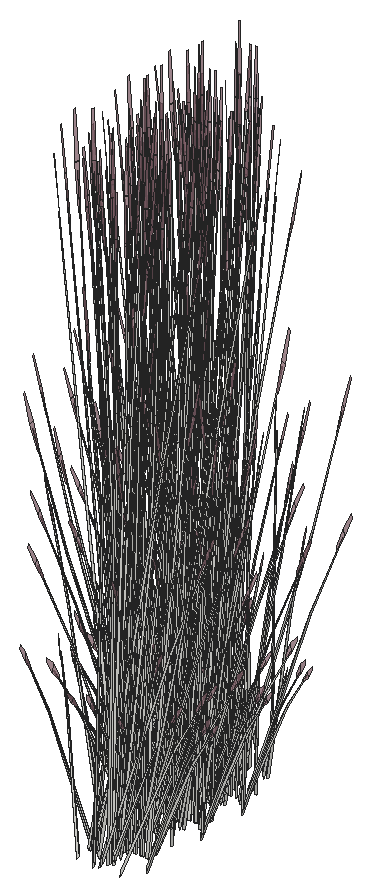
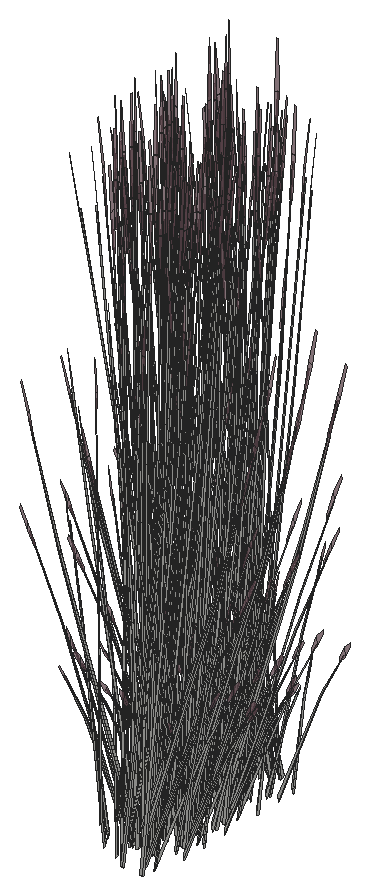
# SketchUp Ruby script. Lengths in inches.
U = 1.inch
M = Sketchup.active_model
def pt(a) = Geom::Point3d.new(a.map { |v| v * U })
def face(e, loops, mat)
  f = e.add_face(loops[0].map { |a| pt(a) })
  loops[1..].each { |l| e.add_face(l.map { |a| pt(a) }).erase! }
  f.material = f.back_material = mat if mat
  f
end
# faces: each face lists its corners as indices into pts; further lists are holes
def faces(e, pts, list, mat = nil) = list.each { |f| face(e, (f[0].is_a?(Array) ? f : [f]).map { |l| l.map { |i| pts[i] } }, mat) }
# xy, xz, yz: faces in a plane at the given z, y or x. An outline is a flat list of corners, or four numbers for a rectangle; further outlines are holes
def ring(l) = l.size == 4 ? [[l[0], l[1]], [l[2], l[1]], [l[2], l[3]], [l[0], l[3]]] : l.each_slice(2).to_a
def flat(e, list, mat, &to3) = list.each { |f| face(e, (f[0].is_a?(Array) ? f : [f]).map { |l| ring(l).map { |u, v| to3.(u, v) } }, mat) }
def xy(e, z, list, mat = nil) = flat(e, list, mat) { |x, y| [x, y, z] }
def xz(e, y, list, mat = nil) = flat(e, list, mat) { |x, z| [x, y, z] }
def yz(e, x, list, mat = nil) = flat(e, list, mat) { |y, z| [x, y, z] }
def lines(e, pts, list) = list.each { |a, b| e.add_line(pt(pts[a]), pt(pts[b])) }
# prism: a flat outline (further loops are holes) pulled along v
def prism(e, loops, v, mat = nil)
  f = face(e, loops, mat); d = Geom::Vector3d.new(v.map { |x| x * U })
  f.pushpull(f.normal.samedirection?(d) ? d.length : -d.length)
end
def box(e, o, s, mat = nil) = prism(e, [[o, [o[0] + s[0], o[1], o[2]], [o[0] + s[0], o[1] + s[1], o[2]], [o[0], o[1] + s[1], o[2]]]], [0, 0, s[2]], mat)
def at(x, y, z, deg = 0) = Geom::Transformation.translation(pt([x, y, z])) * Geom::Transformation.rotation(ORIGIN, Z_AXIS, deg.degrees)
def axes(o, x, y, z) = Geom::Transformation.new([*x, 0, *y, 0, *z, 0, *pt(o).to_a, 1])
def part(name) = M.definitions.add(name)
# library, detail: a bought-in or finely detailed component or shape, given as its bounding box
def library(name, o, s) = part(name).tap { |d| box(d.entities, o, s) }
def detail(e, o, s) = box(e.add_group.entities, o, s)
def put(e, d, t, mat = nil) = e.add_instance(d, t).tap { |i| i.material = mat if mat }
def group(e, t, mat = nil) = e.add_group.tap { |g| g.transformation = t; g.material = mat if mat }.entities
root = M.entities
M.materials.add("LightPink_Translucent").color = [144, 107, 117]
M.materials["LightPink_Translucent"].alpha = 0.75
c1 = part("blade")
p = [[2.15,0.21,22],[0,0.17,0],[0.09,0.45,0],[2.18,0.31,22],[2.29,0.31,22],[0.38,0.45,0],
  [2.48,0.24,33],[2.49,0.24,33],[2.48,0.22,33]]
faces(c1.entities,p,[[0,1,2,3],[4,5,2,3],[6,3,4,7],[8,0,3,6]])
c2 = part("seeds")
p = [[0.3,-0.1,1.38],[-0.01,-0.03,1.59],[-0.01,-0.03,0.03],[0.14,-0.07,-0.07],[0.29,-0.03,3],[0.15,0.01,3.11]]
faces(c2.entities,p,[[0,1,2,3],[1,0,4,5]],"LightPink_Translucent")
c3 = part("blade with seeds")
put(c3.entities,c1,at(0,0,0))
put(c3.entities,c2,axes([2.4,0.25,30.99],[1.5799,-0.05474,1.17369],[-0.12525,1.92788,0.29478],[-0.07173,-0.02425,1.56792]))
put(root,c3,axes([430.05,458.625,152.09],[-0.38354,-0.23583,0.41945],[0.22925,-0.42288,0],[0.08735,0.05371,1.33059]))
put(root,c3,axes([430.8,460.28,154.21],[0.3601,-0.20831,-0.60019],[0.20068,0.4288,0.07243],[0.17399,-0.04871,0.84903]))
put(root,c3,axes([429.18,459.54,151.99],[-0.33979,0.42804,0.38653],[-0.40368,-0.37784,0.15168],[0.08192,-0.04272,1.34202]))
put(root,c3,axes([429.56,460.31,151.94],[-0.38118,-0.40596,-0.0518],[0.38142,-0.40621,0],[-0.01331,-0.01418,1.48322]))
put(root,c3,axes([428.59,458.84,152.09],[-0.11838,0.46875,0.14904],[-0.43321,-0.13265,0.29641],[0.07483,-0.00228,1.35512]))
put(root,c3,axes([428.42,459.21,151.35],[-0.40337,0.18883,1.08919],[-0.12839,-0.54182,0.42321],[0.24769,0.00901,1.23883]))
put(root,c3,axes([429.5,459.36,152.21],[0.07906,-0.42093,0.12232],[0.38625,0.07307,-0.3493],[0.07029,0.04322,1.07074]))
put(root,c3,axes([429.76,458.01,151.97],[0.51304,0.1533,0.25983],[-0.12835,0.54797,-0.30828],[-0.08491,0.06858,1.39295]))
put(root,c3,axes([429.88,463.28,152.1875],[-0.11649,0.09547,1.20808],[-0.34886,-0.1671,-0.25981],[0.06467,-0.20781,0.51652]))
put(root,c3,axes([428.83,460.36,151.99],[0.51796,0.09937,0.38653],[-0.10541,0.56124,0.15168],[-0.07569,-0.05419,1.34202]))
put(root,c3,axes([431.57,459.95,151.26],[-0.02142,-0.07161,1.48974],[0.14855,-0.41887,-0.22758],[0.14984,-0.00603,0.25375]))
put(root,c3,axes([429.35,463.61,154.21],[-0.19559,-0.38351,-0.60019],[0.40262,-0.21373,0.07243],[-0.04574,-0.1853,0.84903]))
put(root,c3,axes([427.14,459.875,151.26],[0.01039,0.07433,1.48974],[-0.20952,0.38819,-0.22758],[-0.14882,-0.01957,0.25375]))
put(root,c3,axes([429.33,459.47,152.3],[-0.24618,-0.39589,0.37796],[0.37289,-0.27878,-0.1819],[0.07967,0.04899,1.2135]))
put(root,c3,axes([428.08,463.1,152.1875],[-0.02482,0.15429,1.20808],[-0.36278,0.12916,-0.25981],[-0.0848,-0.19943,0.51652]))
put(root,c3,axes([430.42,457.97,152.34],[-0.23074,-0.13562,0.97034],[0.29794,-0.1378,0.71294],[0.08036,0.11673,0.21373]))
put(root,c3,axes([429.02,462.76,151.26],[-0.06874,0.01699,1.48974],[-0.38012,-0.19128,-0.22758],[0.00638,-0.15955,0.25375]))
put(root,c3,axes([428.55,461.25,152.09],[0.44036,-0.12519,0.14904],[0.10874,0.46588,0.29641],[-0.03927,-0.06788,1.35512]))
put(root,c3,axes([429.46,459.49,152.25],[0.41376,-0.31314,-0.2458],[0.27514,0.44246,-0.42242],[0.10209,0.04493,1.34921]))
put(root,c3,axes([430.17,463.99,154.21],[0.01066,-0.43628,-0.60019],[0.44902,0.0293,0.07243],[0.04739,-0.18483,0.84903]))
put(root,c3,axes([429.78,460.01,151.86],[0.45849,0,0],[0,0.4883,0],[0,0,1.50718]))
put(root,c3,axes([430.08,458.31,152],[0.25622,0.47263,0],[-0.42866,0.26357,-0.43598],[-0.09763,0.06003,1.38303]))
put(root,c3,axes([429,460.62,152.25],[-0.41376,0.31314,-0.2458],[-0.27514,-0.44246,-0.42242],[-0.10209,-0.04493,1.34921]))
put(root,c3,axes([429.91,458.86,152.09],[-0.44036,0.12519,0.14904],[-0.10874,-0.46588,0.29641],[0.03927,0.06788,1.35512]))
put(root,c3,axes([430.48,458.47,151.26],[0.02986,-0.06809,1.48974],[0.37589,-0.20055,-0.22758],[0.11396,0.1038,0.25375]))
put(root,c3,axes([429.86,456.4375,152.4],[-0.01119,-0.44408,1.19347],[0.50665,0.11511,0.50532],[-0.11983,0.243,1.12654]))
put(root,c3,axes([427.03,458.41,151.26],[0.05497,0.04712,1.48974],[0.09321,0.43661,-0.22758],[-0.12183,0.0931,0.25375]))
put(root,c3,axes([429.46,462.52,152.34],[0.05257,0.27504,0.97034],[-0.29163,-0.15233,0.71294],[0.03138,-0.14083,0.21373]))
put(root,c3,axes([429.63,459.76,152.01],[-0.51796,-0.09937,0.41563],[0.10541,-0.56124,0.1631],[0.07569,0.05419,1.44303]))
put(root,c3,axes([430.46,458.58,152.25],[-0.26279,-0.01479,0.88755],[0.17355,-0.31417,0.49003],[0.10382,0.11162,0.6962]))
put(root,c3,axes([429.21,461.14,151.86],[-0.13371,-0.40664,0],[0.38182,-0.1424,0],[0,0,1.30413]))
put(root,c3,axes([428.96,460.76,152.21],[-0.07906,0.42093,0.12232],[-0.38625,-0.07307,-0.3493],[-0.07029,-0.04322,1.07074]))
put(root,c3,axes([429.71,461.09,151.85],[0.43024,-0.16003,-0.16218],[0.15118,0.46099,0.00007],[0.04749,-0.01769,1.46908]))
put(root,c3,axes([429.86,461.28,152.09],[0.11838,-0.46875,0.14904],[0.43321,0.13265,0.29641],[-0.07483,0.00228,1.35512]))
put(root,c3,axes([429.77,460.22,151.87],[0.28606,0.30466,0],[-0.28606,0.30466,0],[0,0,1.42996]))
put(root,c3,axes([430.54,460.08,152.09],[-0.32198,-0.34356,0.14904],[0.32447,-0.33323,0.29641],[-0.03556,0.07016,1.35512]))
put(root,c3,axes([427.96,462.85,152.34],[0.21377,0.16416,0.97034],[-0.31132,0.09868,0.71294],[-0.06661,-0.12616,0.21373]))
put(root,c3,axes([431.83,460.4,152.34],[-0.2532,0.07787,0.97034],[0.11918,-0.32181,0.71294],[0.13432,0.02202,0.21373]))
put(root,c3,axes([428.47,463.72,154.21],[-0.34944,-0.22798,-0.60019],[0.24834,-0.39949,0.07243],[-0.1266,-0.13612,0.84903]))
put(root,c3,axes([429.12,461.33,151.86],[-0.41314,-0.21175,0],[0.19883,-0.43999,0],[0,0,1.37455]))
put(root,c3,axes([429.46,460.76,152.08],[-0.40016,-0.37963,-0.21282],[0.33672,-0.42629,0.46574],[-0.10776,0.04441,1.42109]))
put(root,c3,axes([428.41,461.49,152.09],[0.38354,0.23583,0.41945],[-0.22925,0.42288,0],[-0.08735,-0.05371,1.33059]))
put(root,c3,axes([429.6,457.82,152.1875],[0.00723,-0.15635,1.20808],[0.34559,-0.17464,-0.25981],[0.10668,0.18713,0.51652]))
put(root,c3,axes([429.76,459.86,152.3],[0.19883,-0.425,0.37796],[0.41314,0.20454,-0.1819],[0,0.09797,1.2135]))
put(root,c3,axes([428.03,459.125,152.34],[-0.01061,-0.28045,0.97034],[0.26501,0.20003,0.71294],[-0.05212,0.13367,0.21373]))
put(root,c3,axes([429.68,460.1,151.9375],[0,0.54548,-0.04762],[-0.51243,0,0],[0,0.01714,1.5153]))
put(root,c3,axes([427.79,463.34,151.26],[-0.0397,0.06213,1.48974],[-0.40116,0.13396,-0.22758],[-0.09691,-0.12186,0.25375]))
put(root,c3,axes([428.1875,461.74,152],[-0.25622,0.47263,0],[-0.42866,-0.26357,-0.43598],[-0.09763,-0.06003,1.38303]))
put(root,c3,axes([428.73,458.45,151.26],[0.06632,-0.02567,1.48974],[0.39894,0.14126,-0.22758],[0.01167,0.15921,0.25375]))
put(root,c3,axes([430.8,460.1,152.09],[0,-0.47166,0.41945],[0.45849,0,0],[0,0.10742,1.33059]))
put(root,c3,axes([429.66,460.45,152.3],[0.44501,-0.02912,0.37796],[0.04024,0.48332,-0.1819],[-0.07967,0.04899,1.2135]))
put(root,c3,axes([430.7,463.57,151.26],[-0.06134,-0.03716,1.48974],[-0.15755,-0.41512,-0.22758],[0.10629,-0.11265,0.25375]))
put(root,c3,axes([429.93,459.96,152.21],[0.38182,-0.13755,0.12232],[0.13371,0.39278,-0.3493],[0,0.08644,1.07074]))
put(root,c3,axes([427.8125,458.52,152.38],[0.37228,-0.08352,0.05498],[0.08559,0.3365,-0.7291],[-0.0236,0.17034,0.65354]))
put(root,c3,axes([431.35,460.91,152.1875],[-0.0987,-0.116,1.20808],[0.12841,-0.38374,-0.25981],[0.19968,0.05198,0.51652]))
put(root,c3,axes([429.59,461.34,151.86],[0.41314,0.21175,0],[-0.19883,0.43999,0],[0,0,1.47801]))
put(root,c3,axes([430.7,464.74,154.21],[0.21406,-0.37215,-0.60019],[0.37511,0.26448,0.07243],[0.12781,-0.13483,0.84903]))
put(root,c3,axes([428.38,463.66,152],[-0.25622,-0.47263,0],[0.42866,-0.26357,-0.43598],[0.09763,-0.06003,1.38303]))
put(root,c3,axes([429.75,461.8,151.85],[-0.25302,-0.47428,-0.04344],[0.42866,-0.26357,0.43598],[-0.10563,0.04516,1.38235]))
put(root,c3,axes([428.95,463.09,151.8],[-0.28319,0.27058,-0.03288],[-0.25948,-0.29635,-0.1491],[-0.01827,-0.08397,0.4918]))
put(root,c3,axes([429.66,460.66,152.21],[0.30276,0.28338,0.12232],[-0.25254,0.31972,-0.3493],[-0.07029,0.04322,1.07074]))
put(root,c3,axes([430.45,461.15,154.21],[0.40965,0.01136,-0.60019],[-0.02751,0.47821,0.07243],[0.17355,0.05047,0.84903]))
put(root,c3,axes([428.85,458.27,154.21],[0.19559,0.38351,-0.60019],[-0.40262,0.21373,0.07243],[0.04574,0.1853,0.84903]))
put(root,c3,axes([429.99,461.53,152.09],[0.38354,-0.23583,0.41945],[0.22925,0.42288,0],[-0.08735,0.05371,1.33059]))
put(root,c3,axes([429.44,461.16,151.9375],[0.17817,0.54185,-0.05079],[-0.50909,0.18987,0],[0.00622,0.01892,1.45452]))
put(root,c3,axes([427.72,458.875,152.1875],[0.12932,-0.07441,1.20808],[0.31929,0.22435,-0.25981],[-0.09503,0.19413,0.51652]))
put(root,c3,axes([431.01,464.4,152.1875],[-0.1464,-0.01397,1.20808],[-0.14998,-0.37477,-0.25981],[0.17985,-0.10602,0.51652]))
put(root,c3,axes([426.88,460.91,152.1875],[0.14242,0.03872,1.20808],[0.09179,0.39548,-0.25981],[-0.19345,0.07403,0.51652]))
put(root,c3,axes([431.12,460.18,152.01],[0.51243,0,0],[0,0.52715,-0.43598],[0,0.12006,1.38303]))
put(root,c3,axes([430.91,460.45,151.86],[-0.51218,-0.00377,-0.04204],[0,-0.52715,0.42192],[-0.0161,0.12,1.33776]))
put(root,c3,axes([429.8,459.99,152.25],[0.46151,0.22505,-0.2458],[-0.22222,0.475,-0.42242],[0.0145,0.11662,1.34921]))
put(root,c3,axes([431.18,463.71,152.34],[-0.1365,0.2401,0.97034],[-0.11733,-0.32258,0.71294],[0.11274,-0.08083,0.21373]))
put(root,c3,axes([426.58,461.74,152.34],[0.17079,-0.21377,0.97034],[0.06739,0.33841,0.71294],[-0.12342,0.0606,0.21373]))
put(root,c3,axes([429.57,460.55,152.25],[0.04775,0.53819,-0.2458],[-0.49736,0.03254,-0.42242],[-0.08758,0.07169,1.34921]))
put(root,c3,axes([428.89,464.97,152.25],[-0.04775,-0.53819,-0.2458],[0.49736,-0.03254,-0.42242],[0.08758,-0.07169,1.34921]))
put(root,c3,axes([427.54,463.58,151.8],[-0.11822,0.38513,-0.03288],[-0.36385,-0.11847,-0.1491],[-0.05524,-0.06299,0.4918]))
put(root,c3,axes([428.66,465.53,152.25],[-0.46151,-0.22505,-0.2458],[0.22222,-0.475,-0.42242],[-0.0145,-0.11662,1.34921]))
put(root,c3,axes([427.34,465.34,152],[-0.51243,0,0],[0,-0.52715,-0.43598],[0,-0.12006,1.38303]))
put(root,c3,axes([427.43,464.4,152.1875],[0.08001,0.13132,1.20808],[-0.18437,0.35694,-0.25981],[-0.18931,-0.08532,0.51652]))
put(root,c3,axes([429.76,461.56,151.97],[0.51304,0.1533,0.25983],[-0.12835,0.54797,-0.30828],[-0.08491,0.06858,1.39295]))
put(root,c3,axes([427.76,464.28,154.21],[-0.40965,-0.01136,-0.60019],[0.02751,-0.47821,0.07243],[-0.17355,-0.05047,0.84903]))
put(root,c3,axes([430.42,461.51,152.34],[-0.23074,-0.13562,0.97034],[0.29794,-0.1378,0.71294],[0.08036,0.11673,0.21373]))
put(root,c3,axes([427.74,465.2,151.97],[-0.38118,0.39654,0.25983],[-0.38142,-0.39237,-0.30828],[-0.01331,-0.11261,1.39295]))
put(root,c3,axes([429.88,467.33,152.1875],[-0.11649,0.09547,1.20808],[-0.34886,-0.1671,-0.25981],[0.06467,-0.20781,0.51652]))
put(root,c3,axes([430.08,461.86,152],[0.25622,0.47263,0],[-0.42866,0.26357,-0.43598],[-0.09763,0.06003,1.38303]))
put(root,c3,axes([429.35,467.66,154.21],[-0.19559,-0.38351,-0.60019],[0.40262,-0.21373,0.07243],[-0.04574,-0.1853,0.84903]))
put(root,c3,axes([430.48,462.02,151.26],[0.02986,-0.06809,1.48974],[0.37589,-0.20055,-0.22758],[0.11396,0.1038,0.25375]))
put(root,c3,axes([429.86,459.99,152.4],[-0.01119,-0.44408,1.19347],[0.50665,0.11511,0.50532],[-0.11983,0.243,1.12654]))
put(root,c3,axes([428.08,467.15,152.1875],[-0.02482,0.15429,1.20808],[-0.36278,0.12916,-0.25981],[-0.0848,-0.19943,0.51652]))
put(root,c3,axes([427.03,461.96,151.26],[0.05497,0.04712,1.48974],[0.09321,0.43661,-0.22758],[-0.12183,0.0931,0.25375]))
put(root,c3,axes([428.95,465.39,152.06],[0.46174,0.2286,0.2033],[-0.22222,0.475,0.42242],[0,-0.1095,1.35626]))
put(root,c3,axes([428.77,466.03,152.06],[0.10862,-0.55889,-0.19793],[0.515,0.09742,0.43313],[-0.08999,-0.07718,1.32161]))
put(root,c3,axes([429.02,466.8125,151.26],[-0.06874,0.01699,1.48974],[-0.38012,-0.19128,-0.22758],[0.00638,-0.15955,0.25375]))
put(root,c3,axes([426.95,464.79,152.34],[0.26163,-0.03375,0.97034],[-0.16596,0.29737,0.71294],[-0.12929,-0.04461,0.21373]))
put(root,c3,axes([430.46,462.13,152.25],[-0.26279,-0.01479,0.88755],[0.17355,-0.31417,0.49003],[0.10382,0.11162,0.6962]))
put(root,c3,axes([430.17,468.04,154.21],[0.01066,-0.43628,-0.60019],[0.44902,0.0293,0.07243],[0.04739,-0.18483,0.84903]))
put(root,c3,axes([428.8,465.07,152.3],[-0.44501,0.02912,0.37796],[-0.04024,-0.48332,-0.1819],[0.07967,-0.04899,1.2135]))
put(root,c3,axes([427.65,465.42,152.09],[0,0.47166,0.41945],[-0.45849,0,0],[0,-0.10742,1.33059]))
put(root,c3,axes([430.27,463.78,152.01],[0.25622,-0.47263,0],[0.42866,0.26357,-0.43598],[0.09763,0.06003,1.38303]))
put(root,c3,axes([428.79,465.24,151.99],[0.17817,0.52741,0.38653],[-0.50909,0.1834,0.15168],[0.00622,-0.09691,1.34202]))
put(root,c3,axes([429.46,466.57,152.34],[0.05257,0.27504,0.97034],[-0.29163,-0.15233,0.71294],[0.03138,-0.14083,0.21373]))
put(root,c3,axes([431.28,465.65,151.67],[-0.26394,0.0566,1.1961],[-0.04201,-0.45055,0.06846],[0.18486,-0.06819,0.68062]))
put(root,c3,axes([431.76,465.25,151.91],[-0.25407,-0.3016,-0.05481],[0.27826,-0.27635,-0.2485],[0.07884,-0.01946,0.81966]))
put(root,c3,axes([428.7,465.66,152.3],[-0.19883,0.425,0.37796],[-0.41314,-0.20454,-0.1819],[0,-0.09797,1.2135]))
put(root,c3,axes([429.6,461.37,152.1875],[0.00723,-0.15635,1.20808],[0.34559,-0.17464,-0.25981],[0.10668,0.18713,0.51652]))
put(root,c3,axes([429.43,465.29,151.86],[0,-0.54574,0],[0.51243,0,0],[0,0,1.51605]))
put(root,c3,axes([430.05,464.03,152.09],[-0.38354,-0.23583,0.41945],[0.22925,-0.42288,0],[0.08735,0.05371,1.33059]))
put(root,c3,axes([430.8,465.68,154.21],[0.3601,-0.20831,-0.60019],[0.20068,0.4288,0.07243],[0.17399,-0.04871,0.84903]))
put(root,c3,axes([429.18,464.94,151.99],[-0.33979,0.42804,0.38653],[-0.40368,-0.37784,0.15168],[0.08192,-0.04272,1.34202]))
put(root,c3,axes([428.03,462.67,152.34],[-0.01061,-0.28045,0.97034],[0.26501,0.20003,0.71294],[-0.05212,0.13367,0.21373]))
put(root,c3,axes([429.56,465.71,151.94],[-0.38118,-0.40596,-0.0518],[0.38142,-0.40621,0],[-0.01331,-0.01418,1.48322]))
put(root,c3,axes([428.59,464.24,152.09],[-0.11838,0.46875,0.14904],[-0.43321,-0.13265,0.29641],[0.07483,-0.00228,1.35512]))
put(root,c3,axes([427.96,466.9,152.34],[0.21377,0.16416,0.97034],[-0.31132,0.09868,0.71294],[-0.06661,-0.12616,0.21373]))
put(root,c3,axes([428.73,462,151.26],[0.06632,-0.02567,1.48974],[0.39894,0.14126,-0.22758],[0.01167,0.15921,0.25375]))
put(root,c3,axes([428.47,467.77,154.21],[-0.34944,-0.22798,-0.60019],[0.24834,-0.39949,0.07243],[-0.1266,-0.13612,0.84903]))
put(root,c3,axes([428.42,464.62,151.35],[-0.40337,0.18883,1.08919],[-0.12839,-0.54182,0.42321],[0.24769,0.00901,1.23883]))
put(root,c3,axes([429.5,464.76,152.21],[0.07906,-0.42093,0.12232],[0.38625,0.07307,-0.3493],[0.07029,0.04322,1.07074]))
put(root,c3,axes([428.83,465.76,151.99],[0.51796,0.09937,0.38653],[-0.10541,0.56124,0.15168],[-0.07569,-0.05419,1.34202]))
put(root,c3,axes([431.57,465.35,151.26],[-0.02142,-0.07161,1.48974],[0.14855,-0.41887,-0.22758],[0.14984,-0.00603,0.25375]))
put(root,c3,axes([427.8125,462.07,152.38],[0.37228,-0.08352,0.05498],[0.08559,0.3365,-0.7291],[-0.0236,0.17034,0.65354]))
put(root,c3,axes([427.14,465.28,151.26],[0.01039,0.07433,1.48974],[-0.20952,0.38819,-0.22758],[-0.14882,-0.01957,0.25375]))
put(root,c3,axes([429.33,464.87,152.3],[-0.24618,-0.39589,0.37796],[0.37289,-0.27878,-0.1819],[0.07967,0.04899,1.2135]))
put(root,c3,axes([427.79,467.4,151.26],[-0.0397,0.06213,1.48974],[-0.40116,0.13396,-0.22758],[-0.09691,-0.12186,0.25375]))
put(root,c3,axes([428.55,466.66,152.09],[0.44036,-0.12519,0.14904],[0.10874,0.46588,0.29641],[-0.03927,-0.06788,1.35512]))
put(root,c3,axes([429.46,464.9,152.25],[0.41376,-0.31314,-0.2458],[0.27514,0.44246,-0.42242],[0.10209,0.04493,1.34921]))
put(root,c3,axes([430.7,467.625,151.26],[-0.06134,-0.03716,1.48974],[-0.15755,-0.41512,-0.22758],[0.10629,-0.11265,0.25375]))
put(root,c3,axes([429.78,465.41,151.86],[0.45849,0,0],[0,0.4883,0],[0,0,1.50718]))
put(root,c3,axes([429,466.02,152.25],[-0.41376,0.31314,-0.2458],[-0.27514,-0.44246,-0.42242],[-0.10209,-0.04493,1.34921]))
put(root,c3,axes([429.91,464.26,152.09],[-0.44036,0.12519,0.14904],[-0.10874,-0.46588,0.29641],[0.03927,0.06788,1.35512]))
put(root,c3,axes([428.85,461.82,154.21],[0.19559,0.38351,-0.60019],[-0.40262,0.21373,0.07243],[0.04574,0.1853,0.84903]))
put(root,c3,axes([430.7,468.8,154.21],[0.21406,-0.37215,-0.60019],[0.37511,0.26448,0.07243],[0.12781,-0.13483,0.84903]))
put(root,c3,axes([427.72,462.42,152.1875],[0.12932,-0.07441,1.20808],[0.31929,0.22435,-0.25981],[-0.09503,0.19413,0.51652]))
put(root,c3,axes([429.63,465.16,152.01],[-0.51796,-0.09937,0.41563],[0.10541,-0.56124,0.1631],[0.07569,0.05419,1.44303]))
put(root,c3,axes([428.38,467.71,152],[-0.25622,-0.47263,0],[0.42866,-0.26357,-0.43598],[0.09763,-0.06003,1.38303]))
put(root,c3,axes([429.21,466.55,151.86],[-0.13371,-0.40664,0],[0.38182,-0.1424,0],[0,0,1.30413]))
put(root,c3,axes([428.95,467.14,151.8],[-0.28319,0.27058,-0.03288],[-0.25948,-0.29635,-0.1491],[-0.01827,-0.08397,0.4918]))
put(root,c3,axes([428.96,466.16,152.21],[-0.07906,0.42093,0.12232],[-0.38625,-0.07307,-0.3493],[-0.07029,-0.04322,1.07074]))
put(root,c3,axes([429.71,466.49,151.85],[0.43024,-0.16003,-0.16218],[0.15118,0.46099,0.00007],[0.04749,-0.01769,1.46908]))
put(root,c3,axes([429.86,466.68,152.09],[0.11838,-0.46875,0.14904],[0.43321,0.13265,0.29641],[-0.07483,0.00228,1.35512]))
put(root,c3,axes([429.77,465.62,151.87],[0.28606,0.30466,0],[-0.28606,0.30466,0],[0,0,1.42996]))
put(root,c3,axes([430.54,465.49,152.09],[-0.32198,-0.34356,0.14904],[0.32447,-0.33323,0.29641],[-0.03556,0.07016,1.35512]))
put(root,c3,axes([431.83,465.8,152.34],[-0.2532,0.07787,0.97034],[0.11918,-0.32181,0.71294],[0.13432,0.02202,0.21373]))
put(root,c3,axes([429.12,466.73,151.86],[-0.41314,-0.21175,0],[0.19883,-0.43999,0],[0,0,1.37455]))
put(root,c3,axes([429.46,466.17,152.08],[-0.40016,-0.37963,-0.21282],[0.33672,-0.42629,0.46574],[-0.10776,0.04441,1.42109]))
put(root,c3,axes([428.41,466.89,152.09],[0.38354,0.23583,0.41945],[-0.22925,0.42288,0],[-0.08735,-0.05371,1.33059]))
put(root,c3,axes([431.01,468.45,152.1875],[-0.1464,-0.01397,1.20808],[-0.14998,-0.37477,-0.25981],[0.17985,-0.10602,0.51652]))
put(root,c3,axes([429.76,465.26,152.3],[0.19883,-0.425,0.37796],[0.41314,0.20454,-0.1819],[0,0.09797,1.2135]))
put(root,c3,axes([431.18,467.77,152.34],[-0.1365,0.2401,0.97034],[-0.11733,-0.32258,0.71294],[0.11274,-0.08083,0.21373]))
put(root,c3,axes([429.68,465.51,151.9375],[0,0.54548,-0.04762],[-0.51243,0,0],[0,0.01714,1.5153]))
put(root,c3,axes([428.1875,467.14,152],[-0.25622,0.47263,0],[-0.42866,-0.26357,-0.43598],[-0.09763,-0.06003,1.38303]))
put(root,c3,axes([430.8,465.5,152.09],[0,-0.47166,0.41945],[0.45849,0,0],[0,0.10742,1.33059]))
put(root,c3,axes([429.66,465.85,152.3],[0.44501,-0.02912,0.37796],[0.04024,0.48332,-0.1819],[-0.07967,0.04899,1.2135]))
put(root,c3,axes([429.93,465.36,152.21],[0.38182,-0.13755,0.12232],[0.13371,0.39278,-0.3493],[0,0.08644,1.07074]))
put(root,c3,axes([428.89,469.02,152.25],[-0.04775,-0.53819,-0.2458],[0.49736,-0.03254,-0.42242],[0.08758,-0.07169,1.34921]))
put(root,c3,axes([431.35,466.32,152.1875],[-0.0987,-0.116,1.20808],[0.12841,-0.38374,-0.25981],[0.19968,0.05198,0.51652]))
put(root,c3,axes([427.54,467.64,151.8],[-0.11822,0.38513,-0.03288],[-0.36385,-0.11847,-0.1491],[-0.05524,-0.06299,0.4918]))
put(root,c3,axes([428.66,469.58,152.25],[-0.46151,-0.22505,-0.2458],[0.22222,-0.475,-0.42242],[-0.0145,-0.11662,1.34921]))
put(root,c3,axes([427.34,469.39,152],[-0.51243,0,0],[0,-0.52715,-0.43598],[0,-0.12006,1.38303]))
put(root,c3,axes([429.59,466.74,151.86],[0.41314,0.21175,0],[-0.19883,0.43999,0],[0,0,1.47801]))
put(root,c3,axes([427.43,468.45,152.1875],[0.08001,0.13132,1.20808],[-0.18437,0.35694,-0.25981],[-0.18931,-0.08532,0.51652]))
put(root,c3,axes([429.75,467.21,151.85],[-0.25302,-0.47428,-0.04344],[0.42866,-0.26357,0.43598],[-0.10563,0.04516,1.38235]))
put(root,c3,axes([427.76,468.34,154.21],[-0.40965,-0.01136,-0.60019],[0.02751,-0.47821,0.07243],[-0.17355,-0.05047,0.84903]))
put(root,c3,axes([429.66,466.06,152.21],[0.30276,0.28338,0.12232],[-0.25254,0.31972,-0.3493],[-0.07029,0.04322,1.07074]))
put(root,c3,axes([430.45,466.55,154.21],[0.40965,0.01136,-0.60019],[-0.02751,0.47821,0.07243],[0.17355,0.05047,0.84903]))
put(root,c3,axes([429.99,466.93,152.09],[0.38354,-0.23583,0.41945],[0.22925,0.42288,0],[-0.08735,0.05371,1.33059]))
put(root,c3,axes([427.74,469.26,151.97],[-0.38118,0.39654,0.25983],[-0.38142,-0.39237,-0.30828],[-0.01331,-0.11261,1.39295]))
put(root,c3,axes([429.44,466.5625,151.9375],[0.17817,0.54185,-0.05079],[-0.50909,0.18987,0],[0.00622,0.01892,1.45452]))
put(root,c3,axes([426.88,466.3125,152.1875],[0.14242,0.03872,1.20808],[0.09179,0.39548,-0.25981],[-0.19345,0.07403,0.51652]))
put(root,c3,axes([431.12,465.58,152.01],[0.51243,0,0],[0,0.52715,-0.43598],[0,0.12006,1.38303]))
put(root,c3,axes([428.95,469.44,152.06],[0.46174,0.2286,0.2033],[-0.22222,0.475,0.42242],[0,-0.1095,1.35626]))
put(root,c3,axes([428.77,470.08,152.06],[0.10862,-0.55889,-0.19793],[0.515,0.09742,0.43313],[-0.08999,-0.07718,1.32161]))
put(root,c3,axes([430.91,465.85,151.86],[-0.51218,-0.00377,-0.04204],[0,-0.52715,0.42192],[-0.0161,0.12,1.33776]))
put(root,c3,axes([429.8,465.39,152.25],[0.46151,0.22505,-0.2458],[-0.22222,0.475,-0.42242],[0.0145,0.11662,1.34921]))
put(root,c3,axes([429.88,471.66,152.1875],[-0.11649,0.09547,1.20808],[-0.34886,-0.1671,-0.25981],[0.06467,-0.20781,0.51652]))
put(root,c3,axes([426.58,467.14,152.34],[0.17079,-0.21377,0.97034],[0.06739,0.33841,0.71294],[-0.12342,0.0606,0.21373]))
put(root,c3,axes([429.35,471.99,154.21],[-0.19559,-0.38351,-0.60019],[0.40262,-0.21373,0.07243],[-0.04574,-0.1853,0.84903]))
put(root,c3,axes([429.57,465.96,152.25],[0.04775,0.53819,-0.2458],[-0.49736,0.03254,-0.42242],[-0.08758,0.07169,1.34921]))
put(root,c3,axes([426.95,468.85,152.34],[0.26163,-0.03375,0.97034],[-0.16596,0.29737,0.71294],[-0.12929,-0.04461,0.21373]))
put(root,c3,axes([428.08,471.48,152.1875],[-0.02482,0.15429,1.20808],[-0.36278,0.12916,-0.25981],[-0.0848,-0.19943,0.51652]))
put(root,c3,axes([428.8,469.12,152.3],[-0.44501,0.02912,0.37796],[-0.04024,-0.48332,-0.1819],[0.07967,-0.04899,1.2135]))
put(root,c3,axes([427.65,469.47,152.09],[0,0.47166,0.41945],[-0.45849,0,0],[0,-0.10742,1.33059]))
put(root,c3,axes([429.02,471.14,151.26],[-0.06874,0.01699,1.48974],[-0.38012,-0.19128,-0.22758],[0.00638,-0.15955,0.25375]))
put(root,c3,axes([430.27,467.83,152.01],[0.25622,-0.47263,0],[0.42866,0.26357,-0.43598],[0.09763,0.06003,1.38303]))
put(root,c3,axes([428.79,469.3,151.99],[0.17817,0.52741,0.38653],[-0.50909,0.1834,0.15168],[0.00622,-0.09691,1.34202]))
put(root,c3,axes([430.17,472.36,154.21],[0.01066,-0.43628,-0.60019],[0.44902,0.0293,0.07243],[0.04739,-0.18483,0.84903]))
put(root,c3,axes([431.28,469.7,151.67],[-0.26394,0.0566,1.1961],[-0.04201,-0.45055,0.06846],[0.18486,-0.06819,0.68062]))
put(root,c3,axes([431.76,469.3,151.91],[-0.25407,-0.3016,-0.05481],[0.27826,-0.27635,-0.2485],[0.07884,-0.01946,0.81966]))
put(root,c3,axes([428.7,469.71,152.3],[-0.19883,0.425,0.37796],[-0.41314,-0.20454,-0.1819],[0,-0.09797,1.2135]))
put(root,c3,axes([429.76,466.96,151.97],[0.51304,0.1533,0.25983],[-0.12835,0.54797,-0.30828],[-0.08491,0.06858,1.39295]))
put(root,c3,axes([429.43,469.34,151.86],[0,-0.54574,0],[0.51243,0,0],[0,0,1.51605]))
put(root,c3,axes([430.05,468.08,152.09],[-0.38354,-0.23583,0.41945],[0.22925,-0.42288,0],[0.08735,0.05371,1.33059]))
put(root,c3,axes([430.8,469.74,154.21],[0.3601,-0.20831,-0.60019],[0.20068,0.4288,0.07243],[0.17399,-0.04871,0.84903]))
put(root,c3,axes([429.46,470.9,152.34],[0.05257,0.27504,0.97034],[-0.29163,-0.15233,0.71294],[0.03138,-0.14083,0.21373]))
put(root,c3,axes([429.18,469,151.99],[-0.33979,0.42804,0.38653],[-0.40368,-0.37784,0.15168],[0.08192,-0.04272,1.34202]))
put(root,c3,axes([430.42,466.92,152.34],[-0.23074,-0.13562,0.97034],[0.29794,-0.1378,0.71294],[0.08036,0.11673,0.21373]))
put(root,c3,axes([429.56,469.76,151.94],[-0.38118,-0.40596,-0.0518],[0.38142,-0.40621,0],[-0.01331,-0.01418,1.48322]))
put(root,c3,axes([428.59,468.29,152.09],[-0.11838,0.46875,0.14904],[-0.43321,-0.13265,0.29641],[0.07483,-0.00228,1.35512]))
put(root,c3,axes([428.42,468.67,151.35],[-0.40337,0.18883,1.08919],[-0.12839,-0.54182,0.42321],[0.24769,0.00901,1.23883]))
put(root,c3,axes([429.5,468.8125,152.21],[0.07906,-0.42093,0.12232],[0.38625,0.07307,-0.3493],[0.07029,0.04322,1.07074]))
put(root,c3,axes([430.08,467.26,152],[0.25622,0.47263,0],[-0.42866,0.26357,-0.43598],[-0.09763,0.06003,1.38303]))
put(root,c3,axes([428.83,469.8125,151.99],[0.51796,0.09937,0.38653],[-0.10541,0.56124,0.15168],[-0.07569,-0.05419,1.34202]))
put(root,c3,axes([431.57,469.41,151.26],[-0.02142,-0.07161,1.48974],[0.14855,-0.41887,-0.22758],[0.14984,-0.00603,0.25375]))
put(root,c3,axes([430.48,467.42,151.26],[0.02986,-0.06809,1.48974],[0.37589,-0.20055,-0.22758],[0.11396,0.1038,0.25375]))
put(root,c3,axes([427.14,469.33,151.26],[0.01039,0.07433,1.48974],[-0.20952,0.38819,-0.22758],[-0.14882,-0.01957,0.25375]))
put(root,c3,axes([429.86,465.39,152.4],[-0.01119,-0.44408,1.19347],[0.50665,0.11511,0.50532],[-0.11983,0.243,1.12654]))
put(root,c3,axes([429.33,468.92,152.3],[-0.24618,-0.39589,0.37796],[0.37289,-0.27878,-0.1819],[0.07967,0.04899,1.2135]))
put(root,c3,axes([427.96,471.23,152.34],[0.21377,0.16416,0.97034],[-0.31132,0.09868,0.71294],[-0.06661,-0.12616,0.21373]))
put(root,c3,axes([427.03,467.36,151.26],[0.05497,0.04712,1.48974],[0.09321,0.43661,-0.22758],[-0.12183,0.0931,0.25375]))
put(root,c3,axes([428.47,472.1,154.21],[-0.34944,-0.22798,-0.60019],[0.24834,-0.39949,0.07243],[-0.1266,-0.13612,0.84903]))
put(root,c3,axes([428.55,470.71,152.09],[0.44036,-0.12519,0.14904],[0.10874,0.46588,0.29641],[-0.03927,-0.06788,1.35512]))
put(root,c3,axes([429.46,468.95,152.25],[0.41376,-0.31314,-0.2458],[0.27514,0.44246,-0.42242],[0.10209,0.04493,1.34921]))
put(root,c3,axes([430.46,467.53,152.25],[-0.26279,-0.01479,0.88755],[0.17355,-0.31417,0.49003],[0.10382,0.11162,0.6962]))
put(root,c3,axes([429.78,469.46,151.86],[0.45849,0,0],[0,0.4883,0],[0,0,1.50718]))
put(root,c3,axes([429,470.08,152.25],[-0.41376,0.31314,-0.2458],[-0.27514,-0.44246,-0.42242],[-0.10209,-0.04493,1.34921]))
put(root,c3,axes([429.91,468.32,152.09],[-0.44036,0.12519,0.14904],[-0.10874,-0.46588,0.29641],[0.03927,0.06788,1.35512]))
put(root,c3,axes([427.79,471.72,151.26],[-0.0397,0.06213,1.48974],[-0.40116,0.13396,-0.22758],[-0.09691,-0.12186,0.25375]))
put(root,c3,axes([430.7,471.95,151.26],[-0.06134,-0.03716,1.48974],[-0.15755,-0.41512,-0.22758],[0.10629,-0.11265,0.25375]))
put(root,c3,axes([429.6,466.77,152.1875],[0.00723,-0.15635,1.20808],[0.34559,-0.17464,-0.25981],[0.10668,0.18713,0.51652]))
put(root,c3,axes([429.63,469.21,152.01],[-0.51796,-0.09937,0.41563],[0.10541,-0.56124,0.1631],[0.07569,0.05419,1.44303]))
put(root,c3,axes([429.21,470.6,151.86],[-0.13371,-0.40664,0],[0.38182,-0.1424,0],[0,0,1.30413]))
put(root,c3,axes([428.96,470.21,152.21],[-0.07906,0.42093,0.12232],[-0.38625,-0.07307,-0.3493],[-0.07029,-0.04322,1.07074]))
put(root,c3,axes([429.71,470.54,151.85],[0.43024,-0.16003,-0.16218],[0.15118,0.46099,0.00007],[0.04749,-0.01769,1.46908]))
put(root,c3,axes([429.86,470.73,152.09],[0.11838,-0.46875,0.14904],[0.43321,0.13265,0.29641],[-0.07483,0.00228,1.35512]))
put(root,c3,axes([428.03,468.07,152.34],[-0.01061,-0.28045,0.97034],[0.26501,0.20003,0.71294],[-0.05212,0.13367,0.21373]))
put(root,c3,axes([429.77,469.67,151.87],[0.28606,0.30466,0],[-0.28606,0.30466,0],[0,0,1.42996]))
put(root,c3,axes([430.7,473.12,154.21],[0.21406,-0.37215,-0.60019],[0.37511,0.26448,0.07243],[0.12781,-0.13483,0.84903]))
put(root,c3,axes([428.38,472.04,152],[-0.25622,-0.47263,0],[0.42866,-0.26357,-0.43598],[0.09763,-0.06003,1.38303]))
put(root,c3,axes([430.54,469.54,152.09],[-0.32198,-0.34356,0.14904],[0.32447,-0.33323,0.29641],[-0.03556,0.07016,1.35512]))
put(root,c3,axes([428.95,471.47,151.8],[-0.28319,0.27058,-0.03288],[-0.25948,-0.29635,-0.1491],[-0.01827,-0.08397,0.4918]))
put(root,c3,axes([428.73,467.4,151.26],[0.06632,-0.02567,1.48974],[0.39894,0.14126,-0.22758],[0.01167,0.15921,0.25375]))
put(root,c3,axes([431.83,469.85,152.34],[-0.2532,0.07787,0.97034],[0.11918,-0.32181,0.71294],[0.13432,0.02202,0.21373]))
put(root,c3,axes([429.12,470.78,151.86],[-0.41314,-0.21175,0],[0.19883,-0.43999,0],[0,0,1.37455]))
put(root,c3,axes([429.46,470.22,152.08],[-0.40016,-0.37963,-0.21282],[0.33672,-0.42629,0.46574],[-0.10776,0.04441,1.42109]))
put(root,c3,axes([428.41,470.95,152.09],[0.38354,0.23583,0.41945],[-0.22925,0.42288,0],[-0.08735,-0.05371,1.33059]))
put(root,c3,axes([427.8125,467.47,152.38],[0.37228,-0.08352,0.05498],[0.08559,0.3365,-0.7291],[-0.0236,0.17034,0.65354]))
put(root,c3,axes([429.76,469.32,152.3],[0.19883,-0.425,0.37796],[0.41314,0.20454,-0.1819],[0,0.09797,1.2135]))
put(root,c3,axes([429.68,469.56,151.9375],[0,0.54548,-0.04762],[-0.51243,0,0],[0,0.01714,1.5153]))
put(root,c3,axes([428.1875,471.19,152],[-0.25622,0.47263,0],[-0.42866,-0.26357,-0.43598],[-0.09763,-0.06003,1.38303]))
put(root,c3,axes([431.01,472.78,152.1875],[-0.1464,-0.01397,1.20808],[-0.14998,-0.37477,-0.25981],[0.17985,-0.10602,0.51652]))
put(root,c3,axes([430.8,469.55,152.09],[0,-0.47166,0.41945],[0.45849,0,0],[0,0.10742,1.33059]))
put(root,c3,axes([429.66,469.9,152.3],[0.44501,-0.02912,0.37796],[0.04024,0.48332,-0.1819],[-0.07967,0.04899,1.2135]))
put(root,c3,axes([429.93,469.41,152.21],[0.38182,-0.13755,0.12232],[0.13371,0.39278,-0.3493],[0,0.08644,1.07074]))
put(root,c3,axes([431.18,472.09,152.34],[-0.1365,0.2401,0.97034],[-0.11733,-0.32258,0.71294],[0.11274,-0.08083,0.21373]))
put(root,c3,axes([431.35,470.37,152.1875],[-0.0987,-0.116,1.20808],[0.12841,-0.38374,-0.25981],[0.19968,0.05198,0.51652]))
put(root,c3,axes([428.85,467.22,154.21],[0.19559,0.38351,-0.60019],[-0.40262,0.21373,0.07243],[0.04574,0.1853,0.84903]))
put(root,c3,axes([429.59,470.79,151.86],[0.41314,0.21175,0],[-0.19883,0.43999,0],[0,0,1.47801]))
put(root,c3,axes([428.89,473.34,152.25],[-0.04775,-0.53819,-0.2458],[0.49736,-0.03254,-0.42242],[0.08758,-0.07169,1.34921]))
put(root,c3,axes([427.72,467.83,152.1875],[0.12932,-0.07441,1.20808],[0.31929,0.22435,-0.25981],[-0.09503,0.19413,0.51652]))
put(root,c3,axes([429.75,471.26,151.85],[-0.25302,-0.47428,-0.04344],[0.42866,-0.26357,0.43598],[-0.10563,0.04516,1.38235]))
put(root,c3,axes([427.54,471.96,151.8],[-0.11822,0.38513,-0.03288],[-0.36385,-0.11847,-0.1491],[-0.05524,-0.06299,0.4918]))
put(root,c3,axes([429.66,470.11,152.21],[0.30276,0.28338,0.12232],[-0.25254,0.31972,-0.3493],[-0.07029,0.04322,1.07074]))
put(root,c3,axes([428.66,473.91,152.25],[-0.46151,-0.22505,-0.2458],[0.22222,-0.475,-0.42242],[-0.0145,-0.11662,1.34921]))
put(root,c3,axes([427.34,473.72,152],[-0.51243,0,0],[0,-0.52715,-0.43598],[0,-0.12006,1.38303]))
put(root,c3,axes([427.43,472.78,152.1875],[0.08001,0.13132,1.20808],[-0.18437,0.35694,-0.25981],[-0.18931,-0.08532,0.51652]))
put(root,c3,axes([430.45,470.6,154.21],[0.40965,0.01136,-0.60019],[-0.02751,0.47821,0.07243],[0.17355,0.05047,0.84903]))
put(root,c3,axes([427.76,472.66,154.21],[-0.40965,-0.01136,-0.60019],[0.02751,-0.47821,0.07243],[-0.17355,-0.05047,0.84903]))
put(root,c3,axes([429.99,470.99,152.09],[0.38354,-0.23583,0.41945],[0.22925,0.42288,0],[-0.08735,0.05371,1.33059]))
put(root,c3,axes([429.44,470.61,151.9375],[0.17817,0.54185,-0.05079],[-0.50909,0.18987,0],[0.00622,0.01892,1.45452]))
put(root,c3,axes([426.88,470.37,152.1875],[0.14242,0.03872,1.20808],[0.09179,0.39548,-0.25981],[-0.19345,0.07403,0.51652]))
